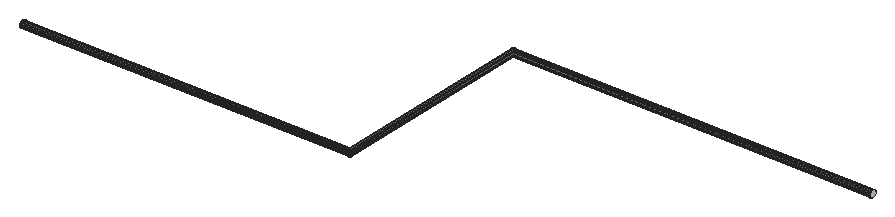
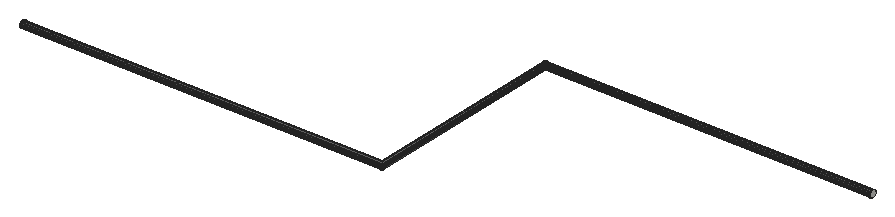
# SketchUp Ruby script. Lengths in inches.
U = 1.inch
M = Sketchup.active_model
def pt(a) = Geom::Point3d.new(a.map { |v| v * U })
def face(e, loops, mat)
  f = e.add_face(loops[0].map { |a| pt(a) })
  loops[1..].each { |l| e.add_face(l.map { |a| pt(a) }).erase! }
  f.material = f.back_material = mat if mat
  f
end
# faces: each face lists its corners as indices into pts; further lists are holes
def faces(e, pts, list, mat = nil) = list.each { |f| face(e, (f[0].is_a?(Array) ? f : [f]).map { |l| l.map { |i| pts[i] } }, mat) }
# xy, xz, yz: faces in a plane at the given z, y or x. An outline is a flat list of corners, or four numbers for a rectangle; further outlines are holes
def ring(l) = l.size == 4 ? [[l[0], l[1]], [l[2], l[1]], [l[2], l[3]], [l[0], l[3]]] : l.each_slice(2).to_a
def flat(e, list, mat, &to3) = list.each { |f| face(e, (f[0].is_a?(Array) ? f : [f]).map { |l| ring(l).map { |u, v| to3.(u, v) } }, mat) }
def xy(e, z, list, mat = nil) = flat(e, list, mat) { |x, y| [x, y, z] }
def xz(e, y, list, mat = nil) = flat(e, list, mat) { |x, z| [x, y, z] }
def yz(e, x, list, mat = nil) = flat(e, list, mat) { |y, z| [x, y, z] }
def lines(e, pts, list) = list.each { |a, b| e.add_line(pt(pts[a]), pt(pts[b])) }
# prism: a flat outline (further loops are holes) pulled along v
def prism(e, loops, v, mat = nil)
  f = face(e, loops, mat); d = Geom::Vector3d.new(v.map { |x| x * U })
  f.pushpull(f.normal.samedirection?(d) ? d.length : -d.length)
end
def box(e, o, s, mat = nil) = prism(e, [[o, [o[0] + s[0], o[1], o[2]], [o[0] + s[0], o[1] + s[1], o[2]], [o[0], o[1] + s[1], o[2]]]], [0, 0, s[2]], mat)
def at(x, y, z, deg = 0) = Geom::Transformation.translation(pt([x, y, z])) * Geom::Transformation.rotation(ORIGIN, Z_AXIS, deg.degrees)
def axes(o, x, y, z) = Geom::Transformation.new([*x, 0, *y, 0, *z, 0, *pt(o).to_a, 1])
def part(name) = M.definitions.add(name)
# library, detail: a bought-in or finely detailed component or shape, given as its bounding box
def library(name, o, s) = part(name).tap { |d| box(d.entities, o, s) }
def detail(e, o, s) = box(e.add_group.entities, o, s)
def put(e, d, t, mat = nil) = e.add_instance(d, t).tap { |i| i.material = mat if mat }
def group(e, t, mat = nil) = e.add_group.tap { |g| g.transformation = t; g.material = mat if mat }.entities
root = M.entities
M.materials.add("[Color M05]").color = [114, 114, 114]
yz(root,18,[[228,292.08,227.74,292.11,227.5,292.21,227.29,292.37,227.13,292.58,227.03,292.82,227,293.08,227.03,293.33,227.13,293.58,227.29,293.78,227.5,293.94,227.74,294.04,228,294.08,228.26,294.04,228.5,293.94,228.71,293.78,228.87,293.58,228.97,293.33,229,293.08,228.97,292.82,228.87,292.58,228.71,292.37,228.5,292.21,228.26,292.11]])
yz(root,231,[[291,292.08,291.26,292.11,291.5,292.21,291.71,292.37,291.87,292.58,291.97,292.82,292,293.08,291.97,293.33,291.87,293.58,291.71,293.78,291.5,293.94,291.26,294.04,291,294.08,290.74,294.04,290.5,293.94,290.29,293.78,290.13,293.58,290.03,293.33,290,293.08,290.03,292.82,290.13,292.58,290.29,292.37,290.5,292.21,290.74,292.11]])
p = [[119.76,227.74,292.11],[120,227.5,292.21],[18,227.5,292.21],[18,227.74,292.11],[119.76,290.74,292.11],[120,290.5,292.21],
  [119.5,228,292.08],[18,228,292.08],[119.5,291,292.08],[119.24,228.26,292.11],[18,228.26,292.11],[119.24,291.26,292.11],
  [119,228.5,292.21],[18,228.5,292.21],[119,291.5,292.21],[231,290.74,292.11],[231,290.5,292.21],[231,291,292.08],
  [231,291.26,292.11],[231,291.5,292.21],[120.21,227.29,292.37],[18,227.29,292.37],[120.21,290.29,292.37],[118.79,228.71,292.37],
  [18,228.71,292.37],[118.79,291.71,292.37],[231,290.29,292.37],[231,291.71,292.37],[120.37,227.13,292.58],[18,227.13,292.58],
  [120.37,290.13,292.58],[118.63,228.87,292.58],[18,228.87,292.58],[118.63,291.87,292.58],[231,290.13,292.58],[231,291.87,292.58],
  [120.47,227.03,292.82],[18,227.03,292.82],[120.47,290.03,292.82],[118.53,228.97,292.82],[18,228.97,292.82],[118.53,291.97,292.82],
  [231,290.03,292.82],[231,291.97,292.82],[120.5,227,293.08],[18,227,293.08],[120.5,290,293.08],[118.5,229,293.08],
  [18,229,293.08],[118.5,292,293.08],[231,290,293.08],[231,292,293.08],[120.47,227.03,293.33],[18,227.03,293.33],
  [120.47,290.03,293.33],[118.53,228.97,293.33],[18,228.97,293.33],[118.53,291.97,293.33],[231,290.03,293.33],[231,291.97,293.33],
  [120.37,227.13,293.58],[18,227.13,293.58],[120.37,290.13,293.58],[118.63,228.87,293.58],[18,228.87,293.58],[118.63,291.87,293.58],
  [231,290.13,293.58],[231,291.87,293.58],[120.21,227.29,293.78],[18,227.29,293.78],[120.21,290.29,293.78],[118.79,228.71,293.78],
  [18,228.71,293.78],[118.79,291.71,293.78],[231,290.29,293.78],[231,291.71,293.78],[120,227.5,293.94],[18,227.5,293.94],
  [120,290.5,293.94],[119,228.5,293.94],[18,228.5,293.94],[119,291.5,293.94],[231,290.5,293.94],[231,291.5,293.94],
  [119.76,227.74,294.04],[18,227.74,294.04],[119.76,290.74,294.04],[119.24,228.26,294.04],[18,228.26,294.04],[119.24,291.26,294.04],
  [231,290.74,294.04],[231,291.26,294.04],[119.5,228,294.08],[18,228,294.08],[119.5,291,294.08],[231,291,294.08]]
faces(root,p,[[0,1,2,3],[4,5,1,0],[6,0,3,7],[8,4,0,6],[9,6,7,10],[11,8,6,9],[12,9,10,13],[14,11,9,12],
  [15,16,5,4],[17,15,4,8],[18,17,8,11],[19,18,11,14],[1,20,21,2],[5,22,20,1],[23,12,13,24],[25,14,12,23],
  [16,26,22,5],[27,19,14,25],[20,28,29,21],[22,30,28,20],[31,23,24,32],[33,25,23,31],[26,34,30,22],[35,27,25,33],
  [28,36,37,29],[30,38,36,28],[39,31,32,40],[41,33,31,39],[34,42,38,30],[43,35,33,41],[36,44,45,37],[38,46,44,36],
  [47,39,40,48],[49,41,39,47],[42,50,46,38],[51,43,41,49],[44,52,53,45],[46,54,52,44],[55,47,48,56],[57,49,47,55],
  [50,58,54,46],[59,51,49,57],[52,60,61,53],[54,62,60,52],[63,55,56,64],[65,57,55,63],[58,66,62,54],[67,59,57,65],
  [60,68,69,61],[62,70,68,60],[71,63,64,72],[73,65,63,71],[66,74,70,62],[75,67,65,73],[68,76,77,69],[70,78,76,68],
  [79,71,72,80],[81,73,71,79],[74,82,78,70],[83,75,73,81],[76,84,85,77],[78,86,84,76],[87,79,80,88],[89,81,79,87],
  [82,90,86,78],[91,83,81,89],[84,92,93,85],[86,94,92,84],[92,87,88,93],[94,89,87,92],[90,95,94,86],[95,91,89,94]],"[Color M05]")
